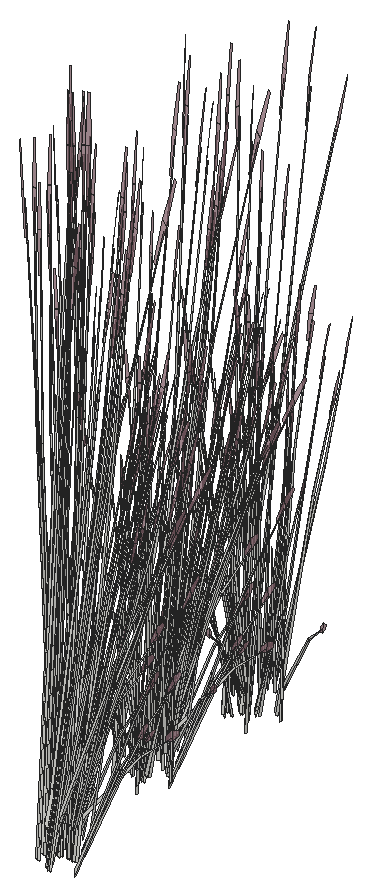
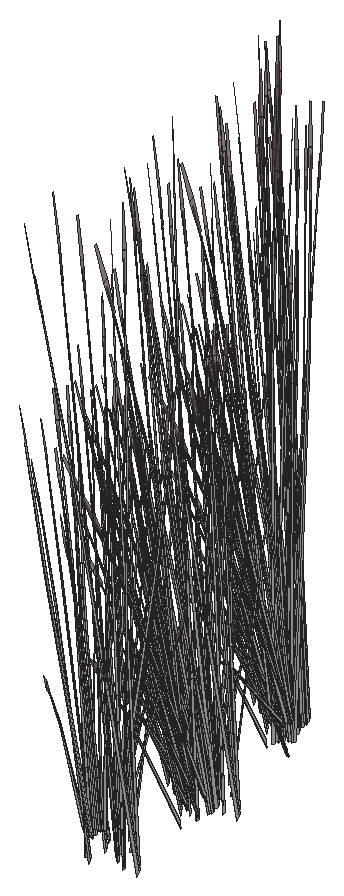
# SketchUp Ruby script. Lengths in inches.
U = 1.inch
M = Sketchup.active_model
def pt(a) = Geom::Point3d.new(a.map { |v| v * U })
def face(e, loops, mat)
  f = e.add_face(loops[0].map { |a| pt(a) })
  loops[1..].each { |l| e.add_face(l.map { |a| pt(a) }).erase! }
  f.material = f.back_material = mat if mat
  f
end
# faces: each face lists its corners as indices into pts; further lists are holes
def faces(e, pts, list, mat = nil) = list.each { |f| face(e, (f[0].is_a?(Array) ? f : [f]).map { |l| l.map { |i| pts[i] } }, mat) }
# xy, xz, yz: faces in a plane at the given z, y or x. An outline is a flat list of corners, or four numbers for a rectangle; further outlines are holes
def ring(l) = l.size == 4 ? [[l[0], l[1]], [l[2], l[1]], [l[2], l[3]], [l[0], l[3]]] : l.each_slice(2).to_a
def flat(e, list, mat, &to3) = list.each { |f| face(e, (f[0].is_a?(Array) ? f : [f]).map { |l| ring(l).map { |u, v| to3.(u, v) } }, mat) }
def xy(e, z, list, mat = nil) = flat(e, list, mat) { |x, y| [x, y, z] }
def xz(e, y, list, mat = nil) = flat(e, list, mat) { |x, z| [x, y, z] }
def yz(e, x, list, mat = nil) = flat(e, list, mat) { |y, z| [x, y, z] }
def lines(e, pts, list) = list.each { |a, b| e.add_line(pt(pts[a]), pt(pts[b])) }
# prism: a flat outline (further loops are holes) pulled along v
def prism(e, loops, v, mat = nil)
  f = face(e, loops, mat); d = Geom::Vector3d.new(v.map { |x| x * U })
  f.pushpull(f.normal.samedirection?(d) ? d.length : -d.length)
end
def box(e, o, s, mat = nil) = prism(e, [[o, [o[0] + s[0], o[1], o[2]], [o[0] + s[0], o[1] + s[1], o[2]], [o[0], o[1] + s[1], o[2]]]], [0, 0, s[2]], mat)
def at(x, y, z, deg = 0) = Geom::Transformation.translation(pt([x, y, z])) * Geom::Transformation.rotation(ORIGIN, Z_AXIS, deg.degrees)
def axes(o, x, y, z) = Geom::Transformation.new([*x, 0, *y, 0, *z, 0, *pt(o).to_a, 1])
def part(name) = M.definitions.add(name)
# library, detail: a bought-in or finely detailed component or shape, given as its bounding box
def library(name, o, s) = part(name).tap { |d| box(d.entities, o, s) }
def detail(e, o, s) = box(e.add_group.entities, o, s)
def put(e, d, t, mat = nil) = e.add_instance(d, t).tap { |i| i.material = mat if mat }
def group(e, t, mat = nil) = e.add_group.tap { |g| g.transformation = t; g.material = mat if mat }.entities
root = M.entities
M.materials.add("LightPink_Translucent").color = [144, 107, 117]
M.materials["LightPink_Translucent"].alpha = 0.75
c1 = part("blade")
p = [[2.15,0.21,22],[0,0.17,0],[0.09,0.45,0],[2.18,0.31,22],[2.29,0.31,22],[0.38,0.45,0],
  [2.48,0.24,33],[2.49,0.24,33],[2.48,0.22,33]]
faces(c1.entities,p,[[0,1,2,3],[4,5,2,3],[6,3,4,7],[8,0,3,6]])
c2 = part("seeds")
p = [[0.3,-0.1,1.38],[-0.01,-0.03,1.59],[-0.01,-0.03,0.03],[0.14,-0.07,-0.07],[0.29,-0.03,3],[0.15,0.01,3.11]]
faces(c2.entities,p,[[0,1,2,3],[1,0,4,5]],"LightPink_Translucent")
c3 = part("blade with seeds")
put(c3.entities,c1,at(0,0,0))
put(c3.entities,c2,axes([2.4,0.25,30.99],[1.5799,-0.05474,1.17369],[-0.12525,1.92788,0.29478],[-0.07173,-0.02425,1.56792]))
put(root,c3,axes([409.98,340.02,-10.61],[-0.02673,-0.08252,1.6421],[0.18538,-0.48271,-0.25086],[0.187,-0.00694,0.2797]))
put(root,c3,axes([407.19,339.47,-9.47],[-0.30722,-0.45622,0.41661],[0.46535,-0.32126,-0.2005],[0.09942,0.05645,1.33761]))
put(root,c3,axes([407.35,339.5,-9.52],[0.51635,-0.36087,-0.27094],[0.34336,0.5099,-0.46562],[0.1274,0.05178,1.4872]))
put(root,c3,axes([409.4,340.45,-7.78],[0.42502,0.15163,-0.32977],[-0.12396,0.44238,0.42575],[0.17112,-0.04056,0.81462]))
put(root,c3,axes([408.65,338.54,-10.12],[0.47863,0.27177,-0.46235],[-0.28609,0.48733,0],[0.10901,0.0619,1.46668]))
put(root,c3,axes([407.74,340.09,-9.95],[0.57217,0,0],[0,0.56272,0],[0,0,1.66132]))
put(root,c3,axes([407.9,338.77,-9.7],[-0.54955,0.14427,0.16428],[-0.1357,-0.53689,0.32672],[0.04901,0.07823,1.49371]))
put(root,c3,axes([408.24,339.9,-8.39],[-0.21212,0.01231,1.59586],[0.14072,-0.53355,0.12904],[0.3023,0.033,0.68222]))
put(root,c3,axes([408.52,338.74,-10.11],[0.12013,0.47362,-0.28847],[-0.47712,0.13449,0.28847],[0.09619,0.05462,1.29413]))
put(root,c3,axes([409.34,340.63,-7.6],[0.18783,0.37061,0.05988],[-0.34252,0.1814,0.47138],[0.15099,-0.03579,0.71878]))
put(root,c3,axes([407.56,339.8,-9.78],[-0.64638,-0.11452,0.45814],[0.13155,-0.64678,0.17978],[0.09446,0.06245,1.59061]))
put(root,c3,axes([409.3,340.5,-7.59],[-0.14449,0.4956,0.447],[-0.47502,-0.16947,0.36857],[0.1868,-0.02978,0.92496]))
put(root,c3,axes([407.04,341.4,-9.95],[-0.16686,-0.46861,0],[0.47648,-0.16411,0],[0,0,1.4375]))
put(root,c3,axes([407.67,341.33,-9.97],[0.53691,-0.18442,-0.17877],[0.18866,0.53125,0.00007],[0.05927,-0.02038,1.61933]))
put(root,c3,axes([407.85,341.55,-9.7],[0.14774,-0.54019,0.16428],[0.54062,0.15287,0.32672],[-0.09339,0.00263,1.49371]))
put(root,c3,axes([407.73,340.33,-9.9375],[0.35699,0.35109,0],[-0.35699,0.35109,0],[0,0,1.57621]))
put(root,c3,axes([408.7,340.18,-9.7],[-0.40181,-0.39593,0.16428],[0.40492,-0.38402,0.32672],[-0.04438,0.08086,1.49371]))
put(root,c3,axes([407.95,339.58,-10.08],[0.53199,0.08911,-0.58063],[-0.11226,0.54969,-0.15239],[0.15876,0.06661,1.28164]))
put(root,c3,axes([410.3,340.54,-9.42],[-0.31598,0.08973,1.06958],[0.14873,-0.37085,0.78586],[0.16763,0.02538,0.23558]))
put(root,c3,axes([406.92,341.61,-9.95],[-0.51557,-0.24403,0],[0.24813,-0.50705,0],[0,0,1.51513]))
put(root,c3,axes([407.72,339.92,-9.47],[0.24813,-0.48978,0.41661],[0.51557,0.23571,-0.2005],[0,0.1129,1.33761]))
put(root,c3,axes([410.16,342.11,-7.62],[-0.04624,-0.04758,1.65179],[0.10116,-0.51007,-0.15608],[0.18215,-0.03259,0.29231]))
put(root,c3,axes([407.63,340.2,-9.87],[0,0.62861,-0.05249],[-0.63949,0,0],[0,0.01975,1.67027]))
put(root,c3,axes([407.68,339.75,-9.94],[0.30722,0.45622,-0.41661],[-0.46535,0.32126,0.2005],[0.09942,0.05645,1.33761]))
put(root,c3,axes([409.75,341.68,-8.34],[-0.09788,-0.45691,-0.03251],[0.46264,-0.10504,-0.14742],[0.09661,0.02897,0.48626]))
put(root,c3,axes([408.55,341.67,-7.3125],[0.02738,-0.55277,-0.11324],[0.51847,0.01511,-0.62851],[0.19968,0.0384,0.95501]))
put(root,c3,axes([409.03,340.19,-9.69],[0,-0.54355,0.46235],[0.57217,0,0],[0,0.1238,1.46668]))
put(root,c3,axes([407.59,340.6,-9.47],[0.55535,-0.03355,0.41661],[0.05022,0.55698,-0.2005],[-0.09942,0.05645,1.33761]))
put(root,c3,axes([407.9375,340.03,-9.5625],[0.47648,-0.15851,0.13483],[0.16686,0.45265,-0.38503],[0,0.09962,1.18024]))
put(root,c3,axes([408.47,341.45,-7.3],[-0.29098,-0.34031,0.32977],[0.33226,-0.32215,-0.42575],[0.16881,0.04902,0.81462]))
put(root,c3,axes([409.71,341.13,-9.59],[-0.12317,-0.13368,1.33163],[0.16025,-0.44223,-0.28638],[0.24919,0.05991,0.56934]))
put(root,c3,axes([407.51,341.62,-9.95],[0.51557,0.24403,0],[-0.24813,0.50705,0],[0,0,1.62917]))
put(root,c3,axes([409,341.34,-7.61],[0.10971,-0.00919,1.62908],[0.30091,-0.42228,-0.25764],[0.19514,0.05574,0.13065]))
put(root,c3,axes([407.6,340.84,-9.5625],[0.37783,0.32657,0.13483],[-0.31516,0.36844,-0.38503],[-0.08772,0.04981,1.18024]))
put(root,c3,axes([408.58,341.4,-7.36],[0.51122,0.01309,-0.66157],[-0.03434,0.5511,0.07984],[0.21658,0.05816,0.93586]))
put(root,c3,axes([408,341.84,-9.69],[0.47863,-0.27177,0.46235],[0.28609,0.48733,0],[-0.10901,0.0619,1.46668]))
put(root,c3,axes([407.32,341.41,-9.87],[0.22235,0.62444,-0.05599],[-0.63531,0.21881,0],[0.00776,0.02181,1.60327]))
put(root,c3,axes([409.41,340.28,-9.79],[0.63949,0,0],[0,0.60749,-0.48057],[0,0.13836,1.52448]))
put(root,c3,axes([409.16,340.6,-9.95],[-0.63917,-0.00435,-0.04634],[0,-0.60749,0.46507],[-0.02009,0.13829,1.47457]))
put(root,c3,axes([407.78,340.07,-9.52],[0.57594,0.25935,-0.27094],[-0.27732,0.5474,-0.46562],[0.0181,0.1344,1.4872]))
put(root,c3,axes([408.89,341.63,-7.78],[0.29098,0.34031,-0.32977],[-0.33226,0.32215,0.42575],[0.16881,0.04902,0.81462]))
put(root,c3,axes([409.03,340.68,-10.11],[-0.35699,0.33913,-0.28847],[-0.35699,-0.33913,0.28847],[0,0.10923,1.29413]))
put(root,c3,axes([408.74,341.76,-7.6],[-0.02575,0.41332,0.05988],[-0.38885,-0.01133,0.47138],[0.14895,0.04325,0.71878]))
put(root,c3,axes([407.71,340.47,-9.94],[-0.24813,0.48978,-0.41661],[-0.51557,-0.23571,0.2005],[0,0.1129,1.33761]))
put(root,c3,axes([408.77,341.63,-7.59],[-0.37709,0.35815,0.447],[-0.32522,-0.38035,0.36857],[0.17692,0.06607,0.92496]))
put(root,c3,axes([407.57,342.04,-7.3],[-0.07899,-0.43781,0.32977],[0.45153,-0.11561,-0.42575],[0.12128,0.12546,0.81462]))
put(root,c3,axes([407.73,341.88,-9.83],[0.64025,0.17667,0.2864],[-0.16018,0.63149,-0.33981],[-0.10597,0.07904,1.53541]))
put(root,c3,axes([409.27,340.7,-10.12],[0,0.54355,-0.46235],[-0.57217,0,0],[0,0.1238,1.46668]))
put(root,c3,axes([407.84,340.76,-8.39],[-0.18996,-0.09365,1.59586],[0.39312,-0.39287,0.12904],[0.24502,0.17723,0.68222]))
put(root,c3,axes([407.88,339.52,-7.83],[-0.44191,-0.28242,1.28769],[0.46662,-0.43971,0.5556],[0.14258,0.26499,1.24467]))
put(root,c3,axes([408.55,341.82,-9.42],[-0.28795,-0.15629,1.06958],[0.37181,-0.1588,0.78586],[0.10029,0.13452,0.23558]))
put(root,c3,axes([407.53,342.27,-7.3125],[0.30474,-0.46525,-0.11324],[0.44133,0.26804,-0.62851],[0.15341,0.13145,0.95501]))
put(root,c3,axes([408.12,342.22,-9.79],[0.31974,0.54466,0],[-0.53494,0.30375,-0.48057],[-0.12184,0.06918,1.52448]))
put(root,c3,axes([407.13,342.66,-7.62],[0.00151,-0.06581,1.65179],[0.43826,-0.29033,-0.15608],[0.15223,0.10363,0.29231]))
put(root,c3,axes([408.625,342.4,-10.61],[0.03726,-0.07847,1.6421],[0.46909,-0.23111,-0.25086],[0.14221,0.11962,0.2797]))
put(root,c3,axes([408.01,340.62,-10.05],[0.18752,0.49766,-0.6445],[-0.54017,0.17923,-0.16915],[0.02073,0.16852,1.42262]))
put(root,c3,axes([407.89,342.04,-7.64],[0.50465,-0.12921,-0.47583],[0.08828,0.48932,-0.36857],[0.13555,0.14022,0.91046]))
put(root,c3,axes([406.49,342.11,-7.3],[0.15418,-0.41799,0.32977],[0.44981,0.12192,-0.42575],[0.04124,0.16829,0.81462]))
put(root,c3,axes([408.59,342.53,-9.52],[-0.32795,-0.01705,0.97832],[0.21658,-0.36206,0.54015],[0.12956,0.12863,0.76741]))
put(root,c3,axes([407.65,342.4375,-7.6],[-0.23243,0.34529,0.05988],[-0.331,-0.20103,0.47138],[0.10701,0.1107,0.71878]))
put(root,c3,axes([407.1,343.6,-6.74],[0.35341,-0.31182,-0.06041],[0.32382,0.34152,-0.27392],[0.0228,0.09677,0.90349]))
put(root,c3,axes([407.74,342.34,-7.59],[-0.50866,0.12474,0.447],[-0.08828,-0.48932,0.36857],[0.11963,0.14421,0.92496]))
put(root,c3,axes([407.52,341.66,-9.59],[0.00902,-0.18018,1.33163],[0.43127,-0.20126,-0.28638],[0.13313,0.21566,0.56934]))
put(root,c3,axes([406.36,342.49,-7.6],[-0.37684,0.18473,0.05988],[-0.18445,-0.33686,0.47138],[0.03639,0.14849,0.71878]))
put(root,c3,axes([406.34,342.29,-7.3125],[0.50045,-0.25306,-0.11324],[0.24593,0.44915,-0.62851],[0.06603,0.18927,0.95501]))
put(root,c3,axes([406.49,342.46,-7.28],[-0.50393,-0.1421,0.49617],[0.17232,-0.46717,0.40911],[0.03028,0.18372,1.0267]))
put(root,c3,axes([406.43,342.39,-10.61],[0.08277,-0.02958,1.6421],[0.49786,0.16279,-0.25086],[0.01456,0.18348,0.2797]))
put(root,c3,axes([406.77,342.27,-7.64],[0.50273,0.13626,-0.47583],[-0.17232,0.46717,-0.36857],[0.0461,0.18809,0.91046]))
put(root,c3,axes([407.06,341.3,-8.39],[-0.1169,-0.17452,1.59586],[0.54019,-0.14692,0.12904],[0.12209,0.27397,0.68222]))
put(root,c3,axes([406.54,342.55,-7.78],[-0.15418,0.41799,-0.32977],[-0.44981,-0.12192,0.42575],[0.04124,0.16829,0.81462]))
put(root,c3,axes([406.59,342.18,-7.36],[0.24409,0.44196,-0.66157],[-0.50245,0.2463,0.07984],[0.05708,0.21354,0.93586]))
put(root,c3,axes([406.23,343.29,-7.61],[0.06483,0.08753,1.62908],[0.52315,0.03439,-0.25764],[0.05261,0.19303,0.13065]))
put(root,c3,axes([405.2,351.16,-9.59],[-0.14537,0.11002,1.33163],[-0.43536,-0.19256,-0.28638],[0.0807,-0.23948,0.56934]))
put(root,c3,axes([405.55,351.98,-7.36],[0.01331,-0.50278,-0.66157],[0.56035,0.03377,0.07984],[0.05914,-0.213,0.93586]))
put(root,c3,axes([406.34,351.19,-7.61],[-0.00494,-0.10818,1.62908],[-0.41695,-0.31265,-0.25764],[0.06446,-0.18952,0.13065]))
put(root,c3,axes([404.92,351.72,-8.39],[-0.09522,0.18683,1.59586],[-0.39947,-0.38663,0.12904],[0.18021,-0.24097,0.68222]))
put(root,c3,axes([405.79,351.67,-7.78],[0.34603,-0.28618,-0.32977],[0.32756,0.32677,0.42575],[0.04984,-0.16603,0.81462]))
put(root,c3,axes([406.22,351.5,-10.61],[-0.07655,-0.04282,1.6421],[-0.19662,-0.47839,-0.25086],[0.13264,-0.12982,0.2797]))
put(root,c3,axes([405.78,351.79,-7.59],[0.36417,0.37086,0.447],[-0.38674,0.31985,0.36857],[0.06718,-0.174,0.92496]))
put(root,c3,axes([405.92,351.82,-7.6],[0.42027,0.02533,0.05988],[-0.01152,0.38243,0.47138],[0.04398,-0.14649,0.71878]))
put(root,c3,axes([406.21,352.85,-7.36],[0.26714,-0.42887,-0.66157],[0.46811,0.30479,0.07984],[0.1595,-0.15539,0.93586]))
put(root,c3,axes([406.2,352.65,-7.64],[-0.13138,-0.49631,-0.47583],[0.49754,-0.08682,-0.36857],[0.14258,-0.13331,0.91046]))
put(root,c3,axes([406.4375,353.01,-7.3125],[-0.47307,-0.29971,-0.11324],[0.27254,-0.43404,-0.62851],[0.13365,-0.15087,0.95501]))
put(root,c3,axes([403.76,351.52,-10.12],[0.47863,-0.27177,-0.46235],[0.28609,0.48733,0],[0.10901,-0.0619,1.46668]))
put(root,c3,axes([406.6,352.46,-9.59],[-0.1827,-0.0161,1.33163],[-0.18717,-0.43188,-0.28638],[0.22444,-0.12218,0.56934]))
put(root,c3,axes([407.6,352.875,-7.62],[-0.0668,-0.00413,1.65179],[-0.27738,-0.44233,-0.15608],[0.11139,-0.14544,0.29231]))
put(root,c3,axes([404.33,352.63,-10.08],[0.34446,-0.40855,-0.58063],[0.42791,0.37046,-0.15239],[0.13803,-0.10191,1.28164]))
put(root,c3,axes([406.8125,351.66,-9.42],[-0.17034,0.27669,1.06958],[-0.14642,-0.37174,0.78586],[0.14069,-0.09315,0.23558]))
put(root,c3,axes([406.57,352.7,-7.78],[0.44516,-0.07768,-0.32977],[0.11755,0.44407,0.42575],[0.12757,-0.11927,0.81462]))
put(root,c3,axes([406.21,352.97,-7.3],[-0.44516,0.07768,0.32977],[-0.11755,-0.44407,-0.42575],[0.12757,-0.11927,0.81462]))
put(root,c3,axes([403.875,351.73,-10.11],[0.47712,0.13449,-0.28847],[-0.12013,0.47362,0.28847],[0.09619,-0.05462,1.29413]))
put(root,c3,axes([406.61,352.9,-7.6],[0.35109,0.22859,0.05988],[-0.2044,0.32553,0.47138],[0.11256,-0.10524,0.71878]))
put(root,c3,axes([406.51,352.8,-7.59],[0.12683,0.50025,0.447],[-0.49754,0.08682,0.36857],[0.14663,-0.11765,0.92496]))
put(root,c3,axes([407.85,353.4,-7.61],[0.07097,-0.08279,1.62908],[-0.09083,-0.50786,-0.25764],[0.17806,-0.09629,0.13065]))
put(root,c3,axes([406.46,354.18,-7.3125],[-0.25732,-0.49218,-0.11324],[0.45669,-0.24187,-0.62851],[0.19245,-0.06494,0.95501]))
put(root,c3,axes([406.43,353.75,-7.64],[0.13855,-0.49442,-0.47583],[0.47502,0.16947,-0.36857],[0.19125,-0.04534,0.91046]))
put(root,c3,axes([405.68,351.74,-9.79],[0.31974,-0.54466,0],[0.53494,0.30375,-0.48057],[0.12184,0.06918,1.52448]))
put(root,c3,axes([406.94,353.89,-10.15],[-0.32938,0.06523,1.31842],[-0.05243,-0.51922,0.07547],[0.2307,-0.07859,0.75023]))
put(root,c3,axes([407.54,353.43,-9.89],[-0.31706,-0.34757,-0.06041],[0.34725,-0.31847,-0.27392],[0.09839,-0.02242,0.90349]))
put(root,c3,axes([405.41,352.02,-9.69],[-0.47863,-0.27177,0.46235],[0.28609,-0.48733,0],[0.10901,0.0619,1.46668]))
put(root,c3,axes([406.34,353.93,-7.36],[0.44939,-0.24006,-0.66157],[0.25044,0.49415,0.07984],[0.21713,-0.05613,0.93586]))
put(root,c3,axes([406.28,354.03,-7.3],[-0.42502,-0.15163,0.32977],[0.12396,-0.44238,-0.42575],[0.17112,-0.04056,0.81462]))
put(root,c3,axes([403.37,352.71,-10.52],[-0.50338,0.21762,1.20058],[-0.16022,-0.62439,0.4665],[0.30911,0.01039,1.36553]))
put(root,c3,axes([404.72,352.87,-9.5625],[0.09866,-0.48509,0.13483],[0.48202,0.0842,-0.38503],[0.08772,0.04981,1.18024]))
put(root,c3,axes([407.3,353.55,-10.61],[-0.02673,-0.08252,1.6421],[0.18538,-0.48271,-0.25086],[0.187,-0.00694,0.2797]))
put(root,c3,axes([404.67,353.03,-9.52],[0.51635,-0.36087,-0.27094],[0.34336,0.5099,-0.46562],[0.1274,0.05178,1.4872]))
put(root,c3,axes([406.72,353.98,-7.78],[0.42502,0.15163,-0.32977],[-0.12396,0.44238,0.42575],[0.17112,-0.04056,0.81462]))
put(root,c3,axes([405.97,352.07,-10.12],[0.47863,0.27177,-0.46235],[-0.28609,0.48733,0],[0.10901,0.0619,1.46668]))
put(root,c3,axes([405.57,353.43,-8.39],[-0.21212,0.01231,1.59586],[0.14072,-0.53355,0.12904],[0.3023,0.033,0.68222]))
put(root,c3,axes([405.84,352.27,-10.11],[0.12013,0.47362,-0.28847],[-0.47712,0.13449,0.28847],[0.09619,0.05462,1.29413]))
put(root,c3,axes([406.66,354.16,-7.6],[0.18783,0.37061,0.05988],[-0.34252,0.1814,0.47138],[0.15099,-0.03579,0.71878]))
put(root,c3,axes([406.625,354.03,-7.59],[-0.14449,0.4956,0.447],[-0.47502,-0.16947,0.36857],[0.1868,-0.02978,0.92496]))
put(root,c3,axes([404.99,354.86,-9.97],[0.53691,-0.18442,-0.17877],[0.18866,0.53125,0.00007],[0.05927,-0.02038,1.61933]))
put(root,c3,axes([405.27,353.11,-10.08],[0.53199,0.08911,-0.58063],[-0.11226,0.54969,-0.15239],[0.15876,0.06661,1.28164]))
put(root,c3,axes([407.625,354.07,-9.42],[-0.31598,0.08973,1.06958],[0.14873,-0.37085,0.78586],[0.16763,0.02538,0.23558]))
put(root,c3,axes([407.48,355.64,-7.62],[-0.04624,-0.04758,1.65179],[0.10116,-0.51007,-0.15608],[0.18215,-0.03259,0.29231]))
put(root,c3,axes([405,353.28,-9.94],[0.30722,0.45622,-0.41661],[-0.46535,0.32126,0.2005],[0.09942,0.05645,1.33761]))
put(root,c3,axes([407.08,355.21,-8.34],[-0.09788,-0.45691,-0.03251],[0.46264,-0.10504,-0.14742],[0.09661,0.02897,0.48626]))
put(root,c3,axes([405.88,355.2,-7.3125],[0.02738,-0.55277,-0.11324],[0.51847,0.01511,-0.62851],[0.19968,0.0384,0.95501]))
put(root,c3,axes([406.35,353.72,-9.69],[0,-0.54355,0.46235],[0.57217,0,0],[0,0.1238,1.46668]))
put(root,c3,axes([405.8,354.98,-7.3],[-0.29098,-0.34031,0.32977],[0.33226,-0.32215,-0.42575],[0.16881,0.04902,0.81462]))
put(root,c3,axes([407.03,354.66,-9.59],[-0.12317,-0.13368,1.33163],[0.16025,-0.44223,-0.28638],[0.24919,0.05991,0.56934]))
put(root,c3,axes([406.33,354.87,-7.61],[0.10971,-0.00919,1.62908],[0.30091,-0.42228,-0.25764],[0.19514,0.05574,0.13065]))
put(root,c3,axes([405.9,354.93,-7.36],[0.51122,0.01309,-0.66157],[-0.03434,0.5511,0.07984],[0.21658,0.05816,0.93586]))
put(root,c3,axes([406.74,353.8125,-9.79],[0.63949,0,0],[0,0.60749,-0.48057],[0,0.13836,1.52448]))
put(root,c3,axes([406.21,355.16,-7.78],[0.29098,0.34031,-0.32977],[-0.33226,0.32215,0.42575],[0.16881,0.04902,0.81462]))
put(root,c3,axes([406.0625,355.29,-7.6],[-0.02575,0.41332,0.05988],[-0.38885,-0.01133,0.47138],[0.14895,0.04325,0.71878]))
put(root,c3,axes([406.1,355.16,-7.59],[-0.37709,0.35815,0.447],[-0.32522,-0.38035,0.36857],[0.17692,0.06607,0.92496]))
put(root,c3,axes([404.9,355.57,-7.3],[-0.07899,-0.43781,0.32977],[0.45153,-0.11561,-0.42575],[0.12128,0.12546,0.81462]))
put(root,c3,axes([406.59,354.23,-10.12],[0,0.54355,-0.46235],[-0.57217,0,0],[0,0.1238,1.46668]))
put(root,c3,axes([405.16,354.29,-8.39],[-0.18996,-0.09365,1.59586],[0.39312,-0.39287,0.12904],[0.24502,0.17723,0.68222]))
put(root,c3,axes([405.2,353.05,-7.83],[-0.44191,-0.28242,1.28769],[0.46662,-0.43971,0.5556],[0.14258,0.26499,1.24467]))
put(root,c3,axes([405.87,355.35,-9.42],[-0.28795,-0.15629,1.06958],[0.37181,-0.1588,0.78586],[0.10029,0.13452,0.23558]))
put(root,c3,axes([404.86,355.8,-7.3125],[0.30474,-0.46525,-0.11324],[0.44133,0.26804,-0.62851],[0.15341,0.13145,0.95501]))
put(root,c3,axes([404.46,356.1875,-7.62],[0.00151,-0.06581,1.65179],[0.43826,-0.29033,-0.15608],[0.15223,0.10363,0.29231]))
put(root,c3,axes([405.95,355.93,-10.61],[0.03726,-0.07847,1.6421],[0.46909,-0.23111,-0.25086],[0.14221,0.11962,0.2797]))
put(root,c3,axes([405.22,355.57,-7.64],[0.50465,-0.12921,-0.47583],[0.08828,0.48932,-0.36857],[0.13555,0.14022,0.91046]))
put(root,c3,axes([405.72,362.37,-9.59],[-0.14537,0.11002,1.33163],[-0.43536,-0.19256,-0.28638],[0.0807,-0.23948,0.56934]))
put(root,c3,axes([405.91,356.07,-9.52],[-0.32795,-0.01705,0.97832],[0.21658,-0.36206,0.54015],[0.12956,0.12863,0.76741]))
put(root,c3,axes([404.97,355.97,-7.6],[-0.23243,0.34529,0.05988],[-0.331,-0.20103,0.47138],[0.10701,0.1107,0.71878]))
put(root,c3,axes([405.07,355.875,-7.59],[-0.50866,0.12474,0.447],[-0.08828,-0.48932,0.36857],[0.11963,0.14421,0.92496]))
put(root,c3,axes([406.07,363.18,-7.36],[0.01331,-0.50278,-0.66157],[0.56035,0.03377,0.07984],[0.05914,-0.213,0.93586]))
put(root,c3,axes([406.85,362.4,-7.61],[-0.00494,-0.10818,1.62908],[-0.41695,-0.31265,-0.25764],[0.06446,-0.18952,0.13065]))
put(root,c3,axes([405.4375,362.93,-8.39],[-0.09522,0.18683,1.59586],[-0.39947,-0.38663,0.12904],[0.18021,-0.24097,0.68222]))
put(root,c3,axes([406.74,362.01,-7.62],[-0.05194,0.04152,1.65179],[-0.50886,-0.14007,-0.15608],[-0.01842,-0.18118,0.29231]))
put(root,c3,axes([404.84,355.1875,-9.59],[0.00902,-0.18018,1.33163],[0.43127,-0.20126,-0.28638],[0.13313,0.21566,0.56934]))
put(root,c3,axes([405.96,363.01,-7.64],[-0.3661,-0.36521,-0.47583],[0.38674,-0.31985,-0.36857],[0.0557,-0.18556,0.91046]))
put(root,c3,axes([406.34,363.21,-7.3125],[-0.56206,-0.02693,-0.11324],[0.01536,-0.50991,-0.62851],[0.03904,-0.19638,0.95501]))
put(root,c3,axes([404.38,354.83,-8.39],[-0.1169,-0.17452,1.59586],[0.54019,-0.14692,0.12904],[0.12209,0.27397,0.68222]))
put(root,c3,axes([406.3,362.88,-7.78],[0.34603,-0.28618,-0.32977],[0.32756,0.32677,0.42575],[0.04984,-0.16603,0.81462]))
put(root,c3,axes([406.73,362.71,-10.61],[-0.07655,-0.04282,1.6421],[-0.19662,-0.47839,-0.25086],[0.13264,-0.12982,0.2797]))
put(root,c3,axes([406.3,362.99,-7.59],[0.36417,0.37086,0.447],[-0.38674,0.31985,0.36857],[0.06718,-0.174,0.92496]))
put(root,c3,axes([406.43,363.03,-7.6],[0.42027,0.02533,0.05988],[-0.01152,0.38243,0.47138],[0.04398,-0.14649,0.71878]))
put(root,c3,axes([406.12,363.29,-7.3],[-0.34603,0.28618,0.32977],[-0.32756,-0.32677,-0.42575],[0.04984,-0.16603,0.81462]))
put(root,c3,axes([406.73,364.06,-7.36],[0.26714,-0.42887,-0.66157],[0.46811,0.30479,0.07984],[0.1595,-0.15539,0.93586]))
put(root,c3,axes([406.72,363.86,-7.64],[-0.13138,-0.49631,-0.47583],[0.49754,-0.08682,-0.36857],[0.14258,-0.13331,0.91046]))
put(root,c3,axes([406.95,364.21,-7.3125],[-0.47307,-0.29971,-0.11324],[0.27254,-0.43404,-0.62851],[0.13365,-0.15087,0.95501]))
put(root,c3,axes([404.28,362.72,-10.12],[0.47863,-0.27177,-0.46235],[0.28609,0.48733,0],[0.10901,-0.0619,1.46668]))
put(root,c3,axes([407.12,363.66,-9.59],[-0.1827,-0.0161,1.33163],[-0.18717,-0.43188,-0.28638],[0.22444,-0.12218,0.56934]))
put(root,c3,axes([408.12,364.08,-7.62],[-0.0668,-0.00413,1.65179],[-0.27738,-0.44233,-0.15608],[0.11139,-0.14544,0.29231]))
put(root,c3,axes([404.84,363.84,-10.08],[0.34446,-0.40855,-0.58063],[0.42791,0.37046,-0.15239],[0.13803,-0.10191,1.28164]))
put(root,c3,axes([407.33,362.87,-9.42],[-0.17034,0.27669,1.06958],[-0.14642,-0.37174,0.78586],[0.14069,-0.09315,0.23558]))
put(root,c3,axes([407.08,363.91,-7.78],[0.44516,-0.07768,-0.32977],[0.11755,0.44407,0.42575],[0.12757,-0.11927,0.81462]))
put(root,c3,axes([404.47,364.3125,-9.52],[-0.05959,-0.62022,-0.27094],[0.62068,-0.0375,-0.46562],[0.1093,-0.08261,1.4872]))
put(root,c3,axes([406.72,364.17,-7.3],[-0.44516,0.07768,0.32977],[-0.11755,-0.44407,-0.42575],[0.12757,-0.11927,0.81462]))
put(root,c3,axes([404.39,362.9375,-10.11],[0.47712,0.13449,-0.28847],[-0.12013,0.47362,0.28847],[0.09619,-0.05462,1.29413]))
put(root,c3,axes([407.125,364.1,-7.6],[0.35109,0.22859,0.05988],[-0.2044,0.32553,0.47138],[0.11256,-0.10524,0.71878]))
put(root,c3,axes([407.03,364,-7.59],[0.12683,0.50025,0.447],[-0.49754,0.08682,0.36857],[0.14663,-0.11765,0.92496]))
put(root,c3,axes([408.37,364.61,-7.61],[0.07097,-0.08279,1.62908],[-0.09083,-0.50786,-0.25764],[0.17806,-0.09629,0.13065]))
put(root,c3,axes([406.97,365.38,-7.3125],[-0.25732,-0.49218,-0.11324],[0.45669,-0.24187,-0.62851],[0.19245,-0.06494,0.95501]))
put(root,c3,axes([406.95,364.96,-7.64],[0.13855,-0.49442,-0.47583],[0.47502,0.16947,-0.36857],[0.19125,-0.04534,0.91046]))
put(root,c3,axes([406.2,362.94,-9.79],[0.31974,-0.54466,0],[0.53494,0.30375,-0.48057],[0.12184,0.06918,1.52448]))
put(root,c3,axes([407.46,365.1,-10.15],[-0.32938,0.06523,1.31842],[-0.05243,-0.51922,0.07547],[0.2307,-0.07859,0.75023]))
put(root,c3,axes([408.06,364.64,-9.89],[-0.31706,-0.34757,-0.06041],[0.34725,-0.31847,-0.27392],[0.09839,-0.02242,0.90349]))
put(root,c3,axes([405.92,363.23,-9.69],[-0.47863,-0.27177,0.46235],[0.28609,-0.48733,0],[0.10901,0.0619,1.46668]))
put(root,c3,axes([406.86,365.14,-7.36],[0.44939,-0.24006,-0.66157],[0.25044,0.49415,0.07984],[0.21713,-0.05613,0.93586]))
put(root,c3,axes([406.79,365.23,-7.3],[-0.42502,-0.15163,0.32977],[0.12396,-0.44238,-0.42575],[0.17112,-0.04056,0.81462]))
put(root,c3,axes([403.88,363.91,-10.52],[-0.50338,0.21762,1.20058],[-0.16022,-0.62439,0.4665],[0.30911,0.01039,1.36553]))
put(root,c3,axes([405.24,364.07,-9.5625],[0.09866,-0.48509,0.13483],[0.48202,0.0842,-0.38503],[0.08772,0.04981,1.18024]))
